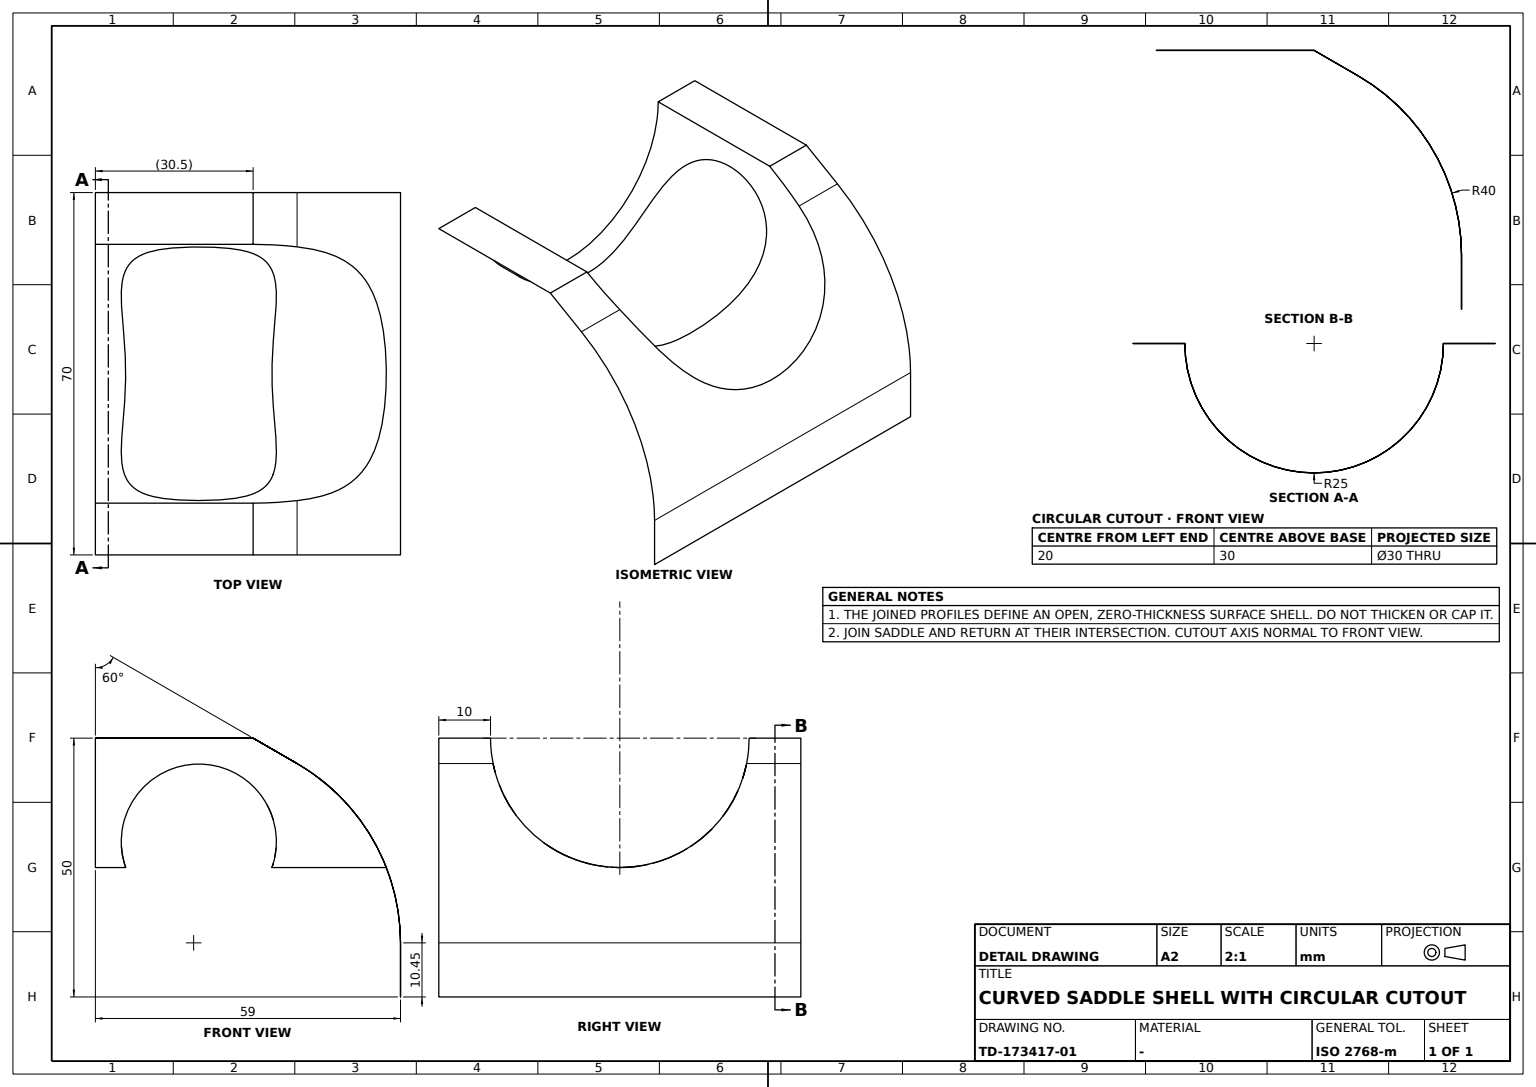
ISO-10303-21;
HEADER;
FILE_DESCRIPTION((''),'2;1');
FILE_NAME('','',(''),(''),'','','');
FILE_SCHEMA(('AUTOMOTIVE_DESIGN'));
ENDSEC;
DATA;
#10=SHAPE_REPRESENTATION_RELATIONSHIP('','',#169,#11);
#11=MANIFOLD_SURFACE_SHAPE_REPRESENTATION('',(#167),#347);
#12=CIRCLE('',#178,40.);
#13=CIRCLE('',#179,40.);
#14=CIRCLE('',#182,25.);
#15=B_SPLINE_CURVE_WITH_KNOTS('',3,(#257,#258,#259,#260,#261,#262,#263,#264,#265,#266,#267,#268,#269,#270,#271,#272,#273,#274,#275,#276,#277,#278,#279,#280),.UNSPECIFIED.,.F.,.F.,(4,1,1,1,1,1,1,1,1,1,1,1,1,1,1,1,1,1,1,1,1,4),(0.,0.00501992959241009,0.0100398591848202,0.0150597887772303,0.0200797183696404,0.0250996479620505,0.0276096127582555,0.0301195775544606,0.0326295423506656,0.0351395071468706,0.0401594367392807,0.0426694015354858,0.0451793663316908,0.0476893311278959,0.0501992959241009,0.055219225516511,0.0602391551089211,0.0627491199051262,0.0652590847013312,0.0702790142937413,0.0752989438861514,0.0803188734785615),.UNSPECIFIED.);
#16=B_SPLINE_CURVE_WITH_KNOTS('',3,(#294,#295,#296,#297,#298,#299,#300,#301,#302,#303,#304,#305,#306,#307,#308,#309,#310,#311,#312,#313,#314,#315,#316,#317,#318,#319,#320,#321,#322,#323,#324,#325,#326,#327,#328,#329,#330),.UNSPECIFIED.,.F.,.F.,(4,1,1,1,1,1,1,1,1,1,1,1,1,1,1,1,1,1,1,1,1,1,1,1,1,1,1,1,1,1,1,1,1,1,4),(0.0624712695147462,0.0665047015541429,0.0705381335935395,0.0745715656329362,0.0786049976723328,0.0826384297117295,0.0866718617511262,0.0907052937905228,0.0947387258299194,0.0987721578693161,0.102805589908713,0.104822305928411,0.106839021948109,0.110872453987506,0.112889170007204,0.114905886026903,0.118939318066299,0.122972750105696,0.127006182145093,0.131039614184489,0.135073046223886,0.139106478263283,0.143139910302679,0.147173342342076,0.151206774381473,0.155240206420869,0.159273638460266,0.163307070499663,0.167340502539059,0.171373934578456,0.175407366617853,0.179440798657249,0.183474230696646,0.187507662736042,0.191541094775439),.UNSPECIFIED.);
#17=B_SPLINE_CURVE_WITH_KNOTS('',3,(#333,#334,#335,#336,#337,#338,#339,#340,#341,#342,#343,#344,#345),.UNSPECIFIED.,.F.,.F.,(4,1,1,1,1,1,1,1,1,1,4),(0.0222340296631745,0.0247488571538978,0.027263684644621,0.0297785121353442,0.0322933396260675,0.0373229946075139,0.0423526495889604,0.0473823045704069,0.0524119595518533,0.0574416145332998,0.0624712695147462),.UNSPECIFIED.);
#18=CYLINDRICAL_SURFACE('',#177,40.);
#19=CYLINDRICAL_SURFACE('',#181,25.);
#20=LINE('',#230,#36);
#21=LINE('',#232,#37);
#22=LINE('',#234,#38);
#23=LINE('',#236,#39);
#24=LINE('',#239,#40);
#25=LINE('',#241,#41);
#26=LINE('',#243,#42);
#27=LINE('',#245,#43);
#28=LINE('',#247,#44);
#29=LINE('',#249,#45);
#30=LINE('',#253,#46);
#31=LINE('',#255,#47);
#32=LINE('',#283,#48);
#33=LINE('',#287,#49);
#34=LINE('',#289,#50);
#35=LINE('',#291,#51);
#36=VECTOR('',#189,1000.);
#37=VECTOR('',#190,1000.);
#38=VECTOR('',#191,1000.);
#39=VECTOR('',#194,1000.);
#40=VECTOR('',#195,1000.);
#41=VECTOR('',#196,1000.);
#42=VECTOR('',#197,1000.);
#43=VECTOR('',#200,1000.);
#44=VECTOR('',#201,1000.);
#45=VECTOR('',#202,1000.);
#46=VECTOR('',#207,1000.);
#47=VECTOR('',#208,1000.);
#48=VECTOR('',#213,1000.);
#49=VECTOR('',#218,1000.);
#50=VECTOR('',#219,1000.);
#51=VECTOR('',#220,1000.);
#52=ORIENTED_EDGE('',*,*,#86,.T.);
#53=ORIENTED_EDGE('',*,*,#87,.T.);
#54=ORIENTED_EDGE('',*,*,#88,.T.);
#55=ORIENTED_EDGE('',*,*,#89,.F.);
#56=ORIENTED_EDGE('',*,*,#90,.T.);
#57=ORIENTED_EDGE('',*,*,#91,.T.);
#58=ORIENTED_EDGE('',*,*,#92,.T.);
#59=ORIENTED_EDGE('',*,*,#93,.T.);
#60=ORIENTED_EDGE('',*,*,#94,.T.);
#61=ORIENTED_EDGE('',*,*,#89,.T.);
#62=ORIENTED_EDGE('',*,*,#95,.T.);
#63=ORIENTED_EDGE('',*,*,#96,.T.);
#64=ORIENTED_EDGE('',*,*,#97,.T.);
#65=ORIENTED_EDGE('',*,*,#93,.F.);
#66=ORIENTED_EDGE('',*,*,#98,.T.);
#67=ORIENTED_EDGE('',*,*,#99,.T.);
#68=ORIENTED_EDGE('',*,*,#100,.T.);
#69=ORIENTED_EDGE('',*,*,#99,.F.);
#70=ORIENTED_EDGE('',*,*,#101,.T.);
#71=ORIENTED_EDGE('',*,*,#102,.T.);
#72=ORIENTED_EDGE('',*,*,#103,.T.);
#73=ORIENTED_EDGE('',*,*,#87,.F.);
#74=ORIENTED_EDGE('',*,*,#104,.T.);
#75=ORIENTED_EDGE('',*,*,#102,.F.);
#76=ORIENTED_EDGE('',*,*,#105,.T.);
#77=ORIENTED_EDGE('',*,*,#106,.T.);
#78=ORIENTED_EDGE('',*,*,#94,.F.);
#79=ORIENTED_EDGE('',*,*,#107,.T.);
#80=ORIENTED_EDGE('',*,*,#90,.F.);
#81=ORIENTED_EDGE('',*,*,#97,.F.);
#82=ORIENTED_EDGE('',*,*,#100,.F.);
#83=ORIENTED_EDGE('',*,*,#86,.F.);
#84=ORIENTED_EDGE('',*,*,#108,.T.);
#85=ORIENTED_EDGE('',*,*,#109,.T.);
#86=EDGE_CURVE('',#110,#111,#128,.F.);
#87=EDGE_CURVE('',#111,#112,#20,.T.);
#88=EDGE_CURVE('',#112,#113,#21,.F.);
#89=EDGE_CURVE('',#110,#113,#22,.T.);
#90=EDGE_CURVE('',#114,#115,#23,.F.);
#91=EDGE_CURVE('',#115,#116,#24,.F.);
#92=EDGE_CURVE('',#116,#117,#25,.T.);
#93=EDGE_CURVE('',#117,#114,#26,.T.);
#94=EDGE_CURVE('',#118,#110,#27,.T.);
#95=EDGE_CURVE('',#113,#119,#28,.F.);
#96=EDGE_CURVE('',#119,#118,#29,.F.);
#97=EDGE_CURVE('',#120,#114,#129,.F.);
#98=EDGE_CURVE('',#117,#121,#30,.T.);
#99=EDGE_CURVE('',#121,#120,#31,.T.);
#100=EDGE_CURVE('',#111,#120,#15,.F.);
#101=EDGE_CURVE('',#121,#122,#12,.T.);
#102=EDGE_CURVE('',#122,#123,#32,.T.);
#103=EDGE_CURVE('',#123,#112,#13,.F.);
#104=EDGE_CURVE('',#124,#123,#33,.F.);
#105=EDGE_CURVE('',#122,#125,#34,.T.);
#106=EDGE_CURVE('',#125,#124,#35,.T.);
#107=EDGE_CURVE('',#118,#115,#14,.T.);
#108=EDGE_CURVE('',#126,#127,#16,.T.);
#109=EDGE_CURVE('',#127,#126,#17,.T.);
#110=VERTEX_POINT('',#228);
#111=VERTEX_POINT('',#229);
#112=VERTEX_POINT('',#231);
#113=VERTEX_POINT('',#233);
#114=VERTEX_POINT('',#237);
#115=VERTEX_POINT('',#238);
#116=VERTEX_POINT('',#240);
#117=VERTEX_POINT('',#242);
#118=VERTEX_POINT('',#246);
#119=VERTEX_POINT('',#248);
#120=VERTEX_POINT('',#252);
#121=VERTEX_POINT('',#254);
#122=VERTEX_POINT('',#282);
#123=VERTEX_POINT('',#284);
#124=VERTEX_POINT('',#288);
#125=VERTEX_POINT('',#290);
#126=VERTEX_POINT('',#331);
#127=VERTEX_POINT('',#332);
#128=ELLIPSE('',#172,50.,25.);
#129=ELLIPSE('',#176,50.,25.);
#130=EDGE_LOOP('',(#52,#53,#54,#55));
#131=EDGE_LOOP('',(#56,#57,#58,#59));
#132=EDGE_LOOP('',(#60,#61,#62,#63));
#133=EDGE_LOOP('',(#64,#65,#66,#67));
#134=EDGE_LOOP('',(#68,#69,#70,#71,#72,#73));
#135=EDGE_LOOP('',(#74,#75,#76,#77));
#136=EDGE_LOOP('',(#78,#79,#80,#81,#82,#83));
#137=EDGE_LOOP('',(#84,#85));
#138=FACE_BOUND('',#130,.T.);
#139=FACE_BOUND('',#131,.T.);
#140=FACE_BOUND('',#132,.T.);
#141=FACE_BOUND('',#133,.T.);
#142=FACE_BOUND('',#134,.T.);
#143=FACE_BOUND('',#135,.T.);
#144=FACE_BOUND('',#136,.T.);
#145=FACE_BOUND('',#137,.T.);
#146=PLANE('',#171);
#147=PLANE('',#173);
#148=PLANE('',#174);
#149=PLANE('',#175);
#150=PLANE('',#180);
#151=ADVANCED_FACE('',(#138),#146,.T.);
#152=ADVANCED_FACE('',(#139),#147,.T.);
#153=ADVANCED_FACE('',(#140),#148,.T.);
#154=ADVANCED_FACE('',(#141),#149,.T.);
#155=ADVANCED_FACE('',(#142),#18,.F.);
#156=ADVANCED_FACE('',(#143),#150,.T.);
#157=ADVANCED_FACE('',(#144,#145),#19,.T.);
#158=OPEN_SHELL('',(#151,#152,#153,#154,#155,#156,#157));
#167=SHELL_BASED_SURFACE_MODEL('',(#158));
#168=SHAPE_DEFINITION_REPRESENTATION(#352,#169);
#169=SHAPE_REPRESENTATION('',(#170),#347);
#170=AXIS2_PLACEMENT_3D('',#225,#183,#184);
#171=AXIS2_PLACEMENT_3D('',#226,#185,#186);
#172=AXIS2_PLACEMENT_3D('',#227,#187,#188);
#173=AXIS2_PLACEMENT_3D('',#235,#192,#193);
#174=AXIS2_PLACEMENT_3D('',#244,#198,#199);
#175=AXIS2_PLACEMENT_3D('',#250,#203,#204);
#176=AXIS2_PLACEMENT_3D('',#251,#205,#206);
#177=AXIS2_PLACEMENT_3D('',#256,#209,#210);
#178=AXIS2_PLACEMENT_3D('',#281,#211,#212);
#179=AXIS2_PLACEMENT_3D('',#285,#214,#215);
#180=AXIS2_PLACEMENT_3D('',#286,#216,#217);
#181=AXIS2_PLACEMENT_3D('',#292,#221,#222);
#182=AXIS2_PLACEMENT_3D('',#293,#223,#224);
#183=DIRECTION('',(0.,0.,1.));
#184=DIRECTION('',(1.,0.,0.));
#185=DIRECTION('',(-0.5,0.,-0.866025403784438));
#186=DIRECTION('',(-0.866025403784438,0.,0.5));
#187=DIRECTION('',(-0.5,0.,-0.866025403784438));
#188=DIRECTION('',(0.866025403784438,0.,-0.5));
#189=DIRECTION('',(0.,-1.,0.));
#190=DIRECTION('',(0.866025403784438,0.,-0.5));
#191=DIRECTION('',(0.,-1.,0.));
#192=DIRECTION('',(0.,0.,-1.));
#193=DIRECTION('',(-1.,0.,0.));
#194=DIRECTION('',(1.,0.,0.));
#195=DIRECTION('',(0.,-1.,0.));
#196=DIRECTION('',(1.,0.,0.));
#197=DIRECTION('',(0.,-1.,0.));
#198=DIRECTION('',(0.,0.,-1.));
#199=DIRECTION('',(-1.,0.,0.));
#200=DIRECTION('',(1.,0.,0.));
#201=DIRECTION('',(1.,0.,0.));
#202=DIRECTION('',(0.,-1.,0.));
#203=DIRECTION('',(-0.5,0.,-0.866025403784438));
#204=DIRECTION('',(-0.866025403784438,0.,0.5));
#205=DIRECTION('',(-0.5,0.,-0.866025403784438));
#206=DIRECTION('',(0.866025403784438,0.,-0.5));
#207=DIRECTION('',(0.866025403784438,0.,-0.5));
#208=DIRECTION('',(0.,-1.,0.));
#209=DIRECTION('',(0.,-1.,0.));
#210=DIRECTION('',(0.,0.,-1.));
#211=DIRECTION('',(0.,1.,0.));
#212=DIRECTION('',(1.,0.,6.12323399573677E-17));
#213=DIRECTION('',(0.,-1.,0.));
#214=DIRECTION('',(0.,1.,0.));
#215=DIRECTION('',(1.,0.,6.12323399573677E-17));
#216=DIRECTION('',(-1.,0.,0.));
#217=DIRECTION('',(0.,0.,1.));
#218=DIRECTION('',(0.,0.,-1.));
#219=DIRECTION('',(0.,0.,-1.));
#220=DIRECTION('',(0.,-1.,0.));
#221=DIRECTION('',(1.,0.,0.));
#222=DIRECTION('',(0.,0.,-1.));
#223=DIRECTION('',(1.,0.,0.));
#224=DIRECTION('',(0.,1.,-6.12323399573677E-17));
#225=CARTESIAN_POINT('',(0.,0.,0.));
#226=CARTESIAN_POINT('',(30.5,35.,0.));
#227=CARTESIAN_POINT('',(30.5,0.,0.));
#228=CARTESIAN_POINT('',(30.5,-25.,-7.65404249467096E-16));
#229=CARTESIAN_POINT('',(39.,-24.5136016665578,-4.90747728811182));
#230=CARTESIAN_POINT('',(39.,35.,-4.90747728811182));
#231=CARTESIAN_POINT('',(39.,-35.,-4.90747728811182));
#232=CARTESIAN_POINT('',(30.5,-35.,0.));
#233=CARTESIAN_POINT('',(30.5,-35.,0.));
#234=CARTESIAN_POINT('',(30.5,35.,0.));
#235=CARTESIAN_POINT('',(0.,35.,0.));
#236=CARTESIAN_POINT('',(0.,25.,0.));
#237=CARTESIAN_POINT('',(30.5,25.,2.29621274840129E-15));
#238=CARTESIAN_POINT('',(0.,25.,-7.65404249467096E-16));
#239=CARTESIAN_POINT('',(0.,35.,0.));
#240=CARTESIAN_POINT('',(0.,35.,0.));
#241=CARTESIAN_POINT('',(0.,35.,0.));
#242=CARTESIAN_POINT('',(30.5,35.,0.));
#243=CARTESIAN_POINT('',(30.5,35.,0.));
#244=CARTESIAN_POINT('',(0.,35.,0.));
#245=CARTESIAN_POINT('',(0.,-25.,0.));
#246=CARTESIAN_POINT('',(0.,-25.,0.));
#247=CARTESIAN_POINT('',(0.,-35.,0.));
#248=CARTESIAN_POINT('',(0.,-35.,0.));
#249=CARTESIAN_POINT('',(0.,35.,0.));
#250=CARTESIAN_POINT('',(30.5,35.,0.));
#251=CARTESIAN_POINT('',(30.5,0.,0.));
#252=CARTESIAN_POINT('',(39.,24.5136016665578,-4.90747728811182));
#253=CARTESIAN_POINT('',(30.5,35.,0.));
#254=CARTESIAN_POINT('',(39.,35.,-4.90747728811182));
#255=CARTESIAN_POINT('',(39.,35.,-4.90747728811182));
#256=CARTESIAN_POINT('',(19.,35.,-39.5484934394894));
#257=CARTESIAN_POINT('',(39.,24.5136016665578,-4.90747728811182));
#258=CARTESIAN_POINT('',(40.4595169294155,24.3449076483174,-5.75012978019668));
#259=CARTESIAN_POINT('',(43.2226916301371,23.8893798729626,-7.58827277541306));
#260=CARTESIAN_POINT('',(46.9512116234846,22.6473975944158,-10.8001978136098));
#261=CARTESIAN_POINT('',(50.0898549211827,20.6887802379828,-14.2469200701005));
#262=CARTESIAN_POINT('',(52.58290176179,17.8512652406453,-17.7019153446755));
#263=CARTESIAN_POINT('',(54.047307212057,14.8552220915512,-20.2226830924747));
#264=CARTESIAN_POINT('',(54.9290737418944,12.0509747228707,-21.9504445954028));
#265=CARTESIAN_POINT('',(55.4343254647612,9.83422357088783,-23.0284806153024));
#266=CARTESIAN_POINT('',(55.8123708528166,7.49838256065673,-23.8936315385352));
#267=CARTESIAN_POINT('',(56.1622457335218,4.21630848135128,-24.7426433680571));
#268=CARTESIAN_POINT('',(56.2929289229427,0.88964544440799,-25.0843539066136));
#269=CARTESIAN_POINT('',(56.2281467006386,-2.51397835217574,-24.9166571227866));
#270=CARTESIAN_POINT('',(56.0777730037697,-4.99765347198075,-24.537566411908));
#271=CARTESIAN_POINT('',(55.8225028296703,-7.42123667929975,-23.9175824112057));
#272=CARTESIAN_POINT('',(55.3156436908665,-10.5851940677611,-22.7561012006132));
#273=CARTESIAN_POINT('',(54.3748732877661,-14.1637280624777,-20.7911973972415));
#274=CARTESIAN_POINT('',(52.882967002132,-17.2370282171949,-18.2193504844615));
#275=CARTESIAN_POINT('',(51.3651102233509,-19.2415716534701,-16.0118915707043));
#276=CARTESIAN_POINT('',(49.5874802553617,-20.9982762594989,-13.697590232112));
#277=CARTESIAN_POINT('',(46.9832990114887,-22.633575090803,-10.8308625991253));
#278=CARTESIAN_POINT('',(43.2340149038326,-23.8882412125179,-7.5951569541188));
#279=CARTESIAN_POINT('',(40.4610263147702,-24.3447331904023,-5.75100122423753));
#280=CARTESIAN_POINT('',(39.,-24.5136016665578,-4.90747728811182));
#281=CARTESIAN_POINT('',(19.,35.,-39.5484934394894));
#282=CARTESIAN_POINT('',(59.,35.,-39.5484934394894));
#283=CARTESIAN_POINT('',(59.,35.,-39.5484934394894));
#284=CARTESIAN_POINT('',(59.,-35.,-39.5484934394894));
#285=CARTESIAN_POINT('',(19.,-35.,-39.5484934394894));
#286=CARTESIAN_POINT('',(59.,35.,-39.5484934394894));
#287=CARTESIAN_POINT('',(59.,-35.,-39.5484934394894));
#288=CARTESIAN_POINT('',(59.,-35.,-50.));
#289=CARTESIAN_POINT('',(59.,35.,-39.5484934394894));
#290=CARTESIAN_POINT('',(59.,35.,-50.));
#291=CARTESIAN_POINT('',(59.,35.,-50.));
#292=CARTESIAN_POINT('',(0.,0.,0.));
#293=CARTESIAN_POINT('',(0.,0.,0.));
#294=CARTESIAN_POINT('',(34.3777802318539,-19.4354930695321,-15.7245543384915));
#295=CARTESIAN_POINT('',(34.6823400595026,-18.6068531518041,-16.7487503208677));
#296=CARTESIAN_POINT('',(35.0279543881029,-16.7288423272529,-18.7260889662853));
#297=CARTESIAN_POINT('',(35.0070213520593,-13.509438641793,-21.1651917534928));
#298=CARTESIAN_POINT('',(34.7116448899926,-9.90098032596683,-23.0755573503144));
#299=CARTESIAN_POINT('',(34.3619730039307,-6.06510033010582,-24.3654843482157));
#300=CARTESIAN_POINT('',(34.1341239290369,-2.05699812939833,-25.0242755346563));
#301=CARTESIAN_POINT('',(34.1315775365332,1.98178481016018,-25.0313320998522));
#302=CARTESIAN_POINT('',(34.3574886885069,6.00941677646821,-24.3792431302806));
#303=CARTESIAN_POINT('',(34.7051020124015,9.8309656151044,-23.1045276990427));
#304=CARTESIAN_POINT('',(35.0022117111842,13.4369689414906,-21.2101021368062));
#305=CARTESIAN_POINT('',(35.0279028747053,16.1111804383968,-19.2006721815));
#306=CARTESIAN_POINT('',(34.7808761698872,18.0786990800923,-17.306693724179));
#307=CARTESIAN_POINT('',(34.3191304932494,19.8364239196843,-15.3171132155351));
#308=CARTESIAN_POINT('',(33.4431782023979,21.3190847389296,-13.1554772156278));
#309=CARTESIAN_POINT('',(32.12166507028,22.4230282821188,-11.0977472003611));
#310=CARTESIAN_POINT('',(30.4593841146123,23.3227159142001,-9.10925356863916));
#311=CARTESIAN_POINT('',(27.8609807992481,24.0283579752727,-7.01265723685481));
#312=CARTESIAN_POINT('',(24.1011581319757,24.4221654786215,-5.37857713688905));
#313=CARTESIAN_POINT('',(20.0306889235455,24.5305171767193,-4.81456840328183));
#314=CARTESIAN_POINT('',(15.9545192329524,24.4251142759161,-5.36332612991625));
#315=CARTESIAN_POINT('',(12.1895990590797,24.037764262773,-6.98052741441752));
#316=CARTESIAN_POINT('',(9.04743743399091,23.1920415900482,-9.50125553852547));
#317=CARTESIAN_POINT('',(6.78449360312081,21.7024034440965,-12.5943201253854));
#318=CARTESIAN_POINT('',(5.47511860225737,19.4983737970811,-15.8165261941946));
#319=CARTESIAN_POINT('',(4.97004203143829,16.702298343458,-18.7517293950753));
#320=CARTESIAN_POINT('',(4.99713535334249,13.4237565091071,-21.2196866576333));
#321=CARTESIAN_POINT('',(5.29275022104653,9.86283349311003,-23.0908996700556));
#322=CARTESIAN_POINT('',(5.64387223122494,5.98582471403903,-24.3855251315327));
#323=CARTESIAN_POINT('',(5.86819586465922,2.00233363308859,-25.0301515066055));
#324=CARTESIAN_POINT('',(5.86502084189664,-2.10108841112702,-25.0215621933628));
#325=CARTESIAN_POINT('',(5.63705687568287,-6.06992491804832,-24.3642024404179));
#326=CARTESIAN_POINT('',(5.2857802434381,-9.93668757105343,-23.0587056647046));
#327=CARTESIAN_POINT('',(4.99374005096582,-13.4828934357668,-21.1818195757172));
#328=CARTESIAN_POINT('',(4.97373698557019,-16.7523227673722,-18.7063929662125));
#329=CARTESIAN_POINT('',(5.31583096443953,-18.6018769125482,-16.7549009348367));
#330=CARTESIAN_POINT('',(5.62221976814614,-19.4354930695321,-15.7245543384915));
#331=CARTESIAN_POINT('',(34.3777802318539,-19.4354930695321,-15.7245543384915));
#332=CARTESIAN_POINT('',(5.62221976814614,-19.4354930695321,-15.7245543384914));
#333=CARTESIAN_POINT('',(5.62221976814615,-19.4354930695321,-15.7245543384914));
#334=CARTESIAN_POINT('',(5.81325186658866,-19.9552491501645,-15.0821376769107));
#335=CARTESIAN_POINT('',(6.29129669316483,-20.9031019406203,-13.7822191222823));
#336=CARTESIAN_POINT('',(7.37930681136366,-22.0858913520456,-11.7832173302154));
#337=CARTESIAN_POINT('',(8.81296127322831,-22.9791763342216,-9.91093969843978));
#338=CARTESIAN_POINT('',(11.2098990798082,-23.848655370626,-7.64688250628913));
#339=CARTESIAN_POINT('',(14.9283404036757,-24.3875082702027,-5.5778736103592));
#340=CARTESIAN_POINT('',(20.0012755234378,-24.5485506850593,-4.71128477277893));
#341=CARTESIAN_POINT('',(25.0680112061844,-24.3876735541544,-5.57698731026539));
#342=CARTESIAN_POINT('',(29.5326889499572,-23.7413335421998,-8.05961544214232));
#343=CARTESIAN_POINT('',(32.8105345436612,-22.2260360219008,-11.7362852227278));
#344=CARTESIAN_POINT('',(33.9979967523457,-20.4687999033443,-14.4473907779257));
#345=CARTESIAN_POINT('',(34.3777802318539,-19.4354930695321,-15.7245543384915));
#347=(GEOMETRIC_REPRESENTATION_CONTEXT(3)GLOBAL_UNCERTAINTY_ASSIGNED_CONTEXT((#348))GLOBAL_UNIT_ASSIGNED_CONTEXT((#351,#350,#349))REPRESENTATION_CONTEXT('export','TOP_LEVEL_ASSEMBLY_PART'));
#348=UNCERTAINTY_MEASURE_WITH_UNIT(LENGTH_MEASURE(0.005),#351,'DISTANCE_ACCURACY_VALUE','Maximum Tolerance applied to model');
#349=(NAMED_UNIT(*)SI_UNIT($,.STERADIAN.)SOLID_ANGLE_UNIT());
#350=(NAMED_UNIT(*)PLANE_ANGLE_UNIT()SI_UNIT($,.RADIAN.));
#351=(LENGTH_UNIT()NAMED_UNIT(*)SI_UNIT(.MILLI.,.METRE.));
#352=PRODUCT_DEFINITION_SHAPE('','',#353);
#353=PRODUCT_DEFINITION('','',#355,#354);
#354=PRODUCT_DEFINITION_CONTEXT('',#361,'design');
#355=PRODUCT_DEFINITION_FORMATION_WITH_SPECIFIED_SOURCE('','',#357,.NOT_KNOWN.);
#356=PRODUCT_RELATED_PRODUCT_CATEGORY('','',(#357));
#357=PRODUCT('','','',(#359));
#358=PRODUCT_CATEGORY('','');
#359=PRODUCT_CONTEXT('',#361,'mechanical');
#360=APPLICATION_PROTOCOL_DEFINITION('international standard','ap242_managed_model_based_3d_engineering',2011,#361);
#361=APPLICATION_CONTEXT('managed model based 3d engineering');
ENDSEC;
END-ISO-10303-21;
